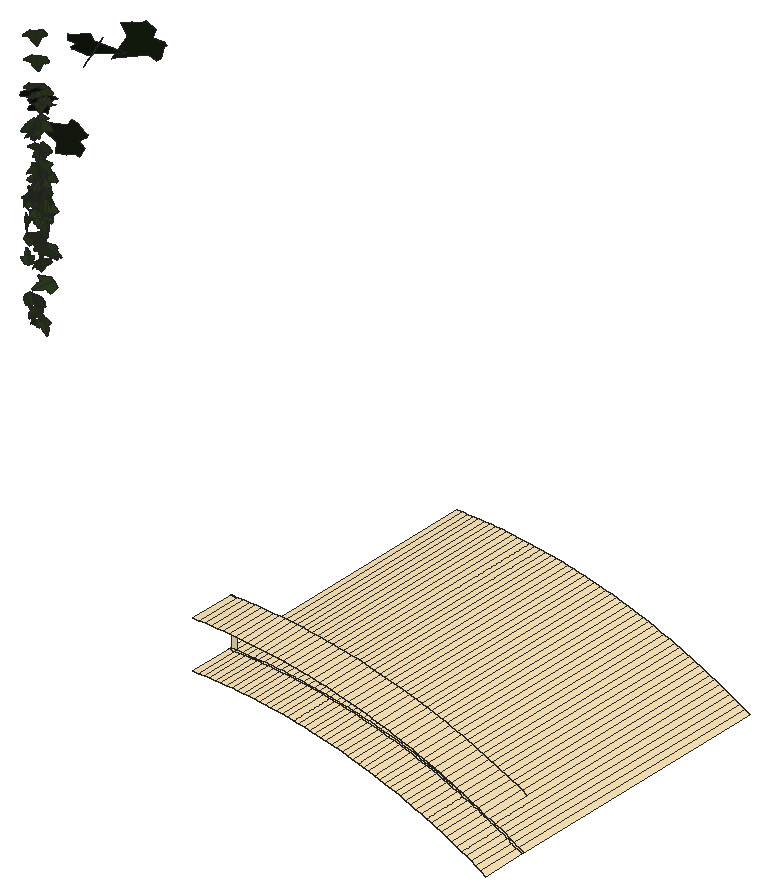
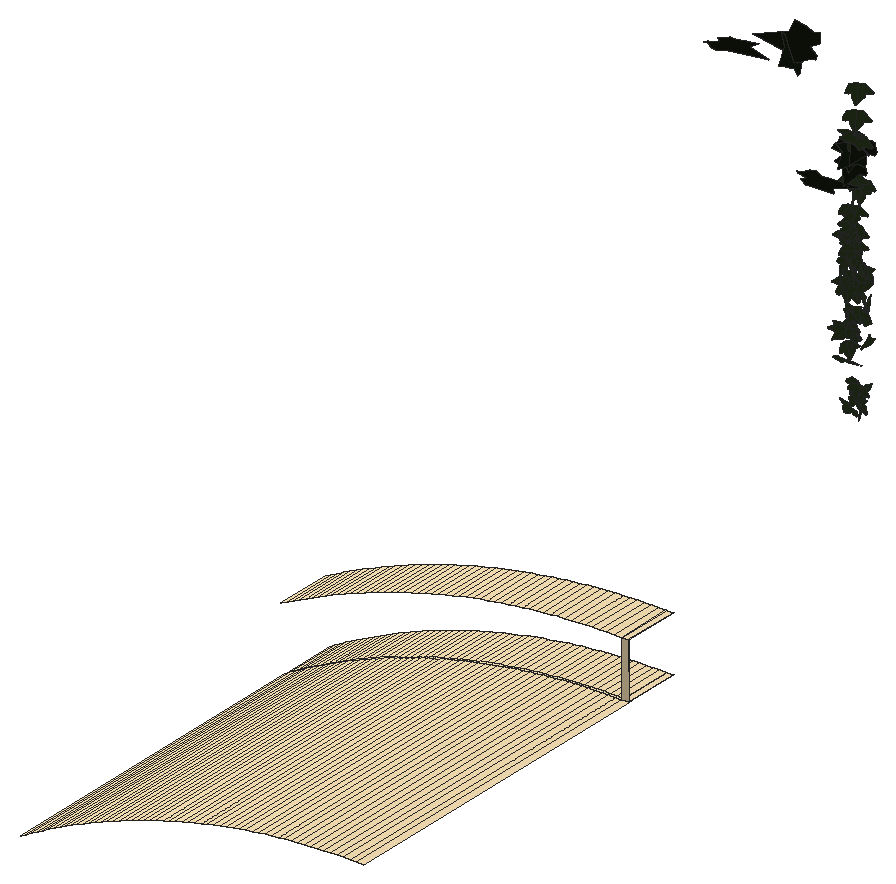
# SketchUp Ruby script. Lengths in inches.
U = 1.inch
M = Sketchup.active_model
def pt(a) = Geom::Point3d.new(a.map { |v| v * U })
def face(e, loops, mat)
  f = e.add_face(loops[0].map { |a| pt(a) })
  loops[1..].each { |l| e.add_face(l.map { |a| pt(a) }).erase! }
  f.material = f.back_material = mat if mat
  f
end
# faces: each face lists its corners as indices into pts; further lists are holes
def faces(e, pts, list, mat = nil) = list.each { |f| face(e, (f[0].is_a?(Array) ? f : [f]).map { |l| l.map { |i| pts[i] } }, mat) }
# xy, xz, yz: faces in a plane at the given z, y or x. An outline is a flat list of corners, or four numbers for a rectangle; further outlines are holes
def ring(l) = l.size == 4 ? [[l[0], l[1]], [l[2], l[1]], [l[2], l[3]], [l[0], l[3]]] : l.each_slice(2).to_a
def flat(e, list, mat, &to3) = list.each { |f| face(e, (f[0].is_a?(Array) ? f : [f]).map { |l| ring(l).map { |u, v| to3.(u, v) } }, mat) }
def xy(e, z, list, mat = nil) = flat(e, list, mat) { |x, y| [x, y, z] }
def xz(e, y, list, mat = nil) = flat(e, list, mat) { |x, z| [x, y, z] }
def yz(e, x, list, mat = nil) = flat(e, list, mat) { |y, z| [x, y, z] }
def lines(e, pts, list) = list.each { |a, b| e.add_line(pt(pts[a]), pt(pts[b])) }
# prism: a flat outline (further loops are holes) pulled along v
def prism(e, loops, v, mat = nil)
  f = face(e, loops, mat); d = Geom::Vector3d.new(v.map { |x| x * U })
  f.pushpull(f.normal.samedirection?(d) ? d.length : -d.length)
end
def box(e, o, s, mat = nil) = prism(e, [[o, [o[0] + s[0], o[1], o[2]], [o[0] + s[0], o[1] + s[1], o[2]], [o[0], o[1] + s[1], o[2]]]], [0, 0, s[2]], mat)
def at(x, y, z, deg = 0) = Geom::Transformation.translation(pt([x, y, z])) * Geom::Transformation.rotation(ORIGIN, Z_AXIS, deg.degrees)
def axes(o, x, y, z) = Geom::Transformation.new([*x, 0, *y, 0, *z, 0, *pt(o).to_a, 1])
def part(name) = M.definitions.add(name)
# library, detail: a bought-in or finely detailed component or shape, given as its bounding box
def library(name, o, s) = part(name).tap { |d| box(d.entities, o, s) }
def detail(e, o, s) = box(e.add_group.entities, o, s)
def put(e, d, t, mat = nil) = e.add_instance(d, t).tap { |i| i.material = mat if mat }
def group(e, t, mat = nil) = e.add_group.tap { |g| g.transformation = t; g.material = mat if mat }.entities
root = M.entities
M.materials.add("1026 AP 7946 SUNNY SIDE UP").color = [254, 231, 186]
M.materials.add("efeu1").color = [18, 25, 13]
M.materials.add("efeu2").color = [43, 57, 29]
c1 = part("ivyleaf_10")
p = [[0,0.5,-0.03],[-0.0625,2.02,-0.43],[-0.19,2.01,-0.46],[-0.54,1.05,-0.29],[-0.52,0.625,-0.18],[-0.83,0.76,-0.28],
  [-1.16,0.64,-0.33],[-1.15,0.33,-0.24],[-0.77,-0.39,0.02],[-0.3,-0.51,0.16],[0.04,-0.48,0.23],[-0.02,2.01,-0.4375],
  [-0.06,2.01,-0.43],[0.04,-0.49,0.23],[0.67,-0.49,0.14],[1.38,0.36,-0.2],[1.375,0.51,-0.24],[0.81,0.65,-0.19],
  [0.62,0.59,-0.15],[0.6,1.09,-0.28],[0.5,1.23,-0.31]]
faces(c1.entities,p,[[0,1,2,3,4,5,6,7,8,9,10],[11,12,0,13,14,15,16,17,18,19,20]],"efeu2")
c2 = part("ivyleaf_9")
p = [[1.54,2.16,1.25],[1.36,2.04,1.19],[-0.21,0.99,0.68],[-0.71,1.11,0.82],[-0.85,0.86,0.67],[-0.8,0.17,0.21],
  [-0.9,-0.01,0.1],[-0.67,-0.16,-0.02],[-0.08,-0.08,-0.05],[-0.03,-0.6,-0.4],[0.65,-0.88,-0.66],[0.83,-0.6,-0.49],
  [1.29,-0.42,-0.43],[1.8125,-0.07,-0.26],[1.21,0.44,0.15]]
faces(c2.entities,p,[[0,1,2,3,4,5,6,7,8,9,10,11,12,13,14]],"efeu1")
xy(root,245.999,[[153.231,213.099,153.236,215],[153.231,215,153.236,215.099]],"1026 AP 7946 SUNNY SIDE UP")
xy(root,246,[[152.978,213.099,153,215,153.002,215,152.981,213.099],[153,215,153,215.099,153.004,215.099,153.002,215],[153,215,153.002,215.099,153.004,215.099,153.002,215]],"1026 AP 7946 SUNNY SIDE UP")
xy(root,247.999,[[153.241,213.099,153.255,215.099]],"1026 AP 7946 SUNNY SIDE UP")
xy(root,248,[[152.988,213.099,153.012,215.099,153.004,215.1,152.981,213.1]],"1026 AP 7946 SUNNY SIDE UP")
xz(root,215.099,[[153.231,245.999,153.004,246,153.012,248,153.241,247.999]],"1026 AP 7946 SUNNY SIDE UP")
p = [[165.136,213.099,242.706],[165.136,215,242.706],[165.338,215,242.585],[165.338,213.099,242.585],[165.136,215.099,242.706],[165.338,215.099,242.585],
  [165.338,227,242.585],[165.136,227,242.706],[164.932,213.099,242.824],[164.932,215,242.824],[164.932,215.099,242.824],[164.932,227,242.824],
  [164.727,213.099,242.94],[164.727,215,242.94],[164.727,215.099,242.94],[164.727,227,242.94],[164.521,213.099,243.054],[164.521,215,243.054],
  [164.521,215.099,243.054],[164.521,227,243.054],[164.314,213.099,243.166],[164.314,215,243.166],[164.314,215.099,243.166],[164.314,227,243.166],
  [164.105,213.099,243.276],[164.105,215,243.276],[164.105,215.099,243.276],[164.105,227,243.276],[163.896,213.099,243.384],[163.896,215,243.384],
  [163.896,215.099,243.384],[163.896,227,243.384],[163.685,213.099,243.49],[163.685,215,243.49],[163.685,215.099,243.49],[163.685,227,243.49],
  [163.474,213.099,243.594],[163.474,215,243.594],[163.474,215.099,243.594],[163.474,227,243.594],[163.261,213.099,243.696],[163.261,215,243.696],
  [163.261,215.099,243.696],[163.261,227,243.696],[163.048,213.099,243.795],[163.048,215,243.795],[163.048,215.099,243.795],[163.048,227,243.795],
  [162.833,213.099,243.893],[162.833,215,243.893],[162.833,215.099,243.893],[162.833,227,243.893],[162.618,213.099,243.989],[162.618,215,243.989],
  [162.618,215.099,243.989],[162.618,227,243.989],[162.402,213.099,244.082],[162.402,215,244.082],[162.402,215.099,244.082],[162.402,227,244.082],
  [162.184,213.099,244.173],[162.184,215,244.173],[162.184,215.099,244.173],[162.184,227,244.173],[161.966,213.099,244.262],[161.966,215,244.262],
  [161.966,215.099,244.262],[161.966,227,244.262],[161.527,213.099,244.434],[161.527,215,244.434],[161.747,215,244.349],[161.747,213.099,244.349],
  [161.527,215.099,244.434],[161.747,215.099,244.349],[161.747,227,244.349],[161.527,227,244.434],[161.307,213.099,244.517],[161.307,215,244.517],
  [161.307,215.099,244.517],[161.307,227,244.517],[161.085,213.099,244.597],[161.085,215,244.597],[161.085,215.099,244.597],[161.085,227,244.597],
  [160.863,213.099,244.675],[160.863,215,244.675],[160.863,215.099,244.675],[160.863,227,244.675],[160.64,213.099,244.751],[160.64,215,244.751],
  [160.64,215.099,244.751],[160.64,227,244.751],[160.192,213.099,244.897],[160.192,215,244.897],[160.416,215,244.825],[160.416,213.099,244.825],
  [165.481,213.099,244.809],[165.481,215.099,244.809],[165.256,215.099,244.93],[165.256,213.099,244.93],[160.192,215.099,244.897],[160.416,215.099,244.825],
  [160.416,227,244.825],[160.192,227,244.897],[159.967,213.099,244.967],[159.967,215,244.967],[165.031,215.099,245.049],[165.031,213.099,245.049],
  [159.967,215.099,244.967],[159.967,227,244.967],[159.515,213.099,245.099],[159.515,215,245.099],[159.741,215,245.034],[159.741,213.099,245.034],
  [164.804,215.099,245.166],[164.804,213.099,245.166],[159.515,215.099,245.099],[159.741,215.099,245.034],[159.741,227,245.034],[159.515,227,245.099],
  [159.287,213.099,245.162],[159.287,215,245.162],[159.287,215.099,245.162],[159.287,227,245.162],[158.832,213.099,245.281],[158.832,215,245.281],
  [159.06,215,245.222],[159.06,213.099,245.222],[164.576,215.099,245.281],[164.576,213.099,245.281],[158.832,215.099,245.281],[159.06,215.099,245.222],
  [159.06,227,245.222],[158.832,227,245.281],[158.373,213.099,245.391],[158.373,215,245.391],[158.603,215,245.337],[158.603,213.099,245.337],
  [164.347,215.099,245.393],[164.347,213.099,245.393],[158.373,215.099,245.391],[158.603,215.099,245.337],[158.603,227,245.337],[158.373,227,245.391],
  [157.913,213.099,245.492],[157.913,215,245.492],[158.143,215,245.442],[158.143,213.099,245.442],[164.116,215.099,245.504],[164.116,213.099,245.504],
  [157.913,215.099,245.492],[158.143,215.099,245.442],[158.143,227,245.442],[157.913,227,245.492],[157.451,213.099,245.584],[157.451,215,245.584],
  [157.682,215,245.539],[157.682,213.099,245.539],[163.885,215.099,245.612],[163.885,213.099,245.612],[157.451,215.099,245.584],[157.682,215.099,245.539],
  [157.682,227,245.539],[157.451,227,245.584],[156.987,213.099,245.667],[156.987,215,245.667],[157.219,215,245.626],[157.219,213.099,245.626],
  [163.653,215.099,245.717],[163.653,213.099,245.717],[156.987,215.099,245.667],[157.219,215.099,245.626],[157.219,227,245.626],[156.987,227,245.667],
  [156.288,213.099,245.774],[156.288,215,245.774],[156.522,215,245.74],[156.522,213.099,245.74],[156.754,215,245.705],[156.754,213.099,245.705],
  [163.419,215.099,245.821],[163.419,213.099,245.821],[156.288,215.099,245.774],[156.522,215.099,245.74],[156.754,215.099,245.705],[156.522,227,245.74],
  [156.288,227,245.774],[156.754,227,245.705],[155.587,213.099,245.86],[155.587,215,245.86],[155.821,215,245.834],[155.821,213.099,245.834],
  [156.055,215,245.805],[156.055,213.099,245.805],[163.185,215.099,245.922],[163.185,213.099,245.922],[155.587,215.099,245.86],[155.821,215.099,245.834],
  [156.055,215.099,245.805],[155.821,227,245.834],[155.587,227,245.86],[156.055,227,245.805],[154.413,213.099,245.958],[154.413,215,245.958],
  [154.648,215,245.943],[154.648,213.099,245.943],[154.883,215,245.926],[154.883,213.099,245.926],[155.118,215,245.906],[155.118,213.099,245.906],
  [155.352,215,245.884],[155.352,213.099,245.884],[162.95,215.099,246.021],[162.95,213.099,246.021],[154.413,215.099,245.958],[154.648,215.099,245.943],
  [154.883,215.099,245.926],[155.118,215.099,245.906],[155.352,215.099,245.884],[154.648,227,245.943],[154.413,227,245.958],[154.883,227,245.926],
  [155.118,227,245.906],[155.352,227,245.884],[152.981,213.099,246],[153.002,215,246],[153.231,215,245.999],[153.231,213.099,245.999],
  [153.236,213.099,245.999],[153.236,215,245.999],[153.471,215,245.995],[153.471,213.099,245.995],[153.707,215,245.99],[153.707,213.099,245.99],
  [153.942,215,245.981],[153.942,213.099,245.981],[154.178,215,245.971],[154.178,213.099,245.971],[162.713,215.099,246.117],[162.713,213.099,246.117],
  [153.004,215.099,246],[153.231,215.099,245.999],[153.236,215.099,245.999],[153.471,215.099,245.995],[153.707,215.099,245.99],[153.942,215.099,245.981],
  [154.178,215.099,245.971],[153.012,215.099,248],[153.002,215.099,246],[153.004,215.1,248],[153.236,227,245.999],[153,215.099,246],
  [153,227,246],[153.471,227,245.995],[153.707,227,245.99],[153.942,227,245.981],[154.178,227,245.971],[162.476,215.099,246.212],
  [162.476,213.099,246.212],[162.238,215.099,246.303],[162.238,213.099,246.303],[161.999,215.099,246.393],[161.999,213.099,246.393],[161.759,215.099,246.48],
  [161.759,213.099,246.48],[161.518,215.099,246.565],[161.518,213.099,246.565],[161.277,213.099,246.647],[161.277,215.099,246.647],[161.034,215.099,246.727],
  [161.034,213.099,246.727],[160.791,215.099,246.805],[160.791,213.099,246.805],[160.547,215.099,246.88],[160.547,213.099,246.88],[160.303,215.099,246.953],
  [160.303,213.099,246.953],[160.057,213.099,247.024],[160.057,215.099,247.024],[159.811,215.099,247.092],[159.811,213.099,247.092],[159.565,215.099,247.158],
  [159.565,213.099,247.158],[159.317,213.099,247.221],[159.317,215.099,247.221],[159.07,215.099,247.282],[159.07,213.099,247.282],[158.821,213.099,247.34],
  [158.821,215.099,247.34],[158.572,215.099,247.396],[158.572,213.099,247.396],[158.322,213.099,247.449],[158.322,215.099,247.449],[158.072,215.099,247.5],
  [158.072,213.099,247.5],[157.822,213.099,247.549],[157.822,215.099,247.549],[157.571,215.099,247.595],[157.571,213.099,247.595],[157.319,213.099,247.639],
  [157.319,215.099,247.639],[157.067,215.099,247.68],[157.067,213.099,247.68],[156.815,213.099,247.719],[156.815,215.099,247.719],[156.5625,215.099,247.755],
  [156.5625,213.099,247.755],[155.802,213.099,247.849],[155.802,215.099,247.849],[155.548,215.099,247.875],[155.548,213.099,247.875],[156.056,213.099,247.82],
  [156.056,215.099,247.82],[156.309,213.099,247.789],[156.309,215.099,247.789],[154.785,213.099,247.939],[154.785,215.099,247.939],[154.531,215.099,247.955],
  [154.531,213.099,247.955],[155.04,213.099,247.92],[155.04,215.099,247.92],[155.294,213.099,247.899],[155.294,215.099,247.899],[153.241,213.099,247.999],
  [153.241,215.099,247.999],[152.988,213.099,248],[153.51,213.099,247.995],[153.51,215.099,247.995],[153.255,215.099,247.999],[153.255,213.099,247.999],
  [153.766,213.099,247.989],[153.766,215.099,247.989],[154.021,213.099,247.98],[154.021,215.099,247.98],[154.276,213.099,247.969],[154.276,215.099,247.969]]
faces(root,p,[[0,1,2,3],[1,4,5,2],[6,5,4,7],[8,9,1,0],[9,10,4,1],[7,4,10,11],[12,13,9,8],[13,14,10,9],
  [11,10,14,15],[16,17,13,12],[17,18,14,13],[15,14,18,19],[20,21,17,16],[21,22,18,17],[19,18,22,23],[24,25,21,20],
  [25,26,22,21],[23,22,26,27],[28,29,25,24],[29,30,26,25],[27,26,30,31],[32,33,29,28],[33,34,30,29],[31,30,34,35],
  [36,37,33,32],[37,38,34,33],[35,34,38,39],[40,41,37,36],[41,42,38,37],[39,38,42,43],[44,45,41,40],[45,46,42,41],
  [43,42,46,47],[48,49,45,44],[49,50,46,45],[47,46,50,51],[52,53,49,48],[53,54,50,49],[51,50,54,55],[56,57,53,52],
  [57,58,54,53],[55,54,58,59],[60,61,57,56],[61,62,58,57],[59,58,62,63],[64,65,61,60],[65,66,62,61],[63,62,66,67],
  [68,69,70,71],[71,70,65,64],[69,72,73,70],[70,73,66,65],[74,73,72,75],[67,66,73,74],[76,77,69,68],[77,78,72,69],
  [75,72,78,79],[80,81,77,76],[81,82,78,77],[79,78,82,83],[84,85,81,80],[85,86,82,81],[83,82,86,87],[88,89,85,84],
  [89,90,86,85],[87,86,90,91],[92,93,94,95],[95,94,89,88],[96,97,98,99],[93,100,101,94],[94,101,90,89],[102,101,100,103],
  [91,90,101,102],[104,105,93,92],[99,98,106,107],[105,108,100,93],[103,100,108,109],[110,111,112,113],[113,112,105,104],[107,106,114,115],
  [111,116,117,112],[112,117,108,105],[118,117,116,119],[109,108,117,118],[120,121,111,110],[121,122,116,111],[119,116,122,123],[124,125,126,127],
  [127,126,121,120],[115,114,128,129],[125,130,131,126],[126,131,122,121],[132,131,130,133],[123,122,131,132],[134,135,136,137],[137,136,125,124],
  [129,128,138,139],[135,140,141,136],[136,141,130,125],[142,141,140,143],[133,130,141,142],[144,145,146,147],[147,146,135,134],[139,138,148,149],
  [145,150,151,146],[146,151,140,135],[152,151,150,153],[143,140,151,152],[154,155,156,157],[157,156,145,144],[149,148,158,159],[155,160,161,156],
  [156,161,150,145],[162,161,160,163],[153,150,161,162],[164,165,166,167],[167,166,155,154],[159,158,168,169],[165,170,171,166],[166,171,160,155],
  [172,171,170,173],[163,160,171,172],[174,175,176,177],[177,176,178,179],[179,178,165,164],[169,168,180,181],[175,182,183,176],[176,183,184,178],
  [178,184,170,165],[185,183,182,186],[187,184,183,185],[173,170,184,187],[188,189,190,191],[191,190,192,193],[193,192,175,174],[181,180,194,195],
  [189,196,197,190],[190,197,198,192],[192,198,182,175],[199,197,196,200],[201,198,197,199],[186,182,198,201],[202,203,204,205],[205,204,206,207],
  [207,206,208,209],[209,208,210,211],[211,210,189,188],[195,194,212,213],[203,214,215,204],[204,215,216,206],[206,216,217,208],[208,217,218,210],
  [210,218,196,189],[219,215,214,220],[221,216,215,219],[222,217,216,221],[223,218,217,222],[200,196,218,223],[224,225,226,227],[228,229,230,231],
  [231,230,232,233],[233,232,234,235],[235,234,236,237],[237,236,203,202],[213,212,238,239],[240,241,226,225],[229,242,243,230],[230,243,244,232],
  [232,244,245,234],[234,245,246,236],[236,246,214,203],[247,240,248,249],[250,242,241,240,248,251,252],[253,243,242,250],[254,244,243,253],[255,245,244,254],
  [256,246,245,255],[220,214,246,256],[239,238,257,258],[258,257,259,260],[260,259,261,262],[262,261,263,264],[264,263,265,266],[267,268,269,270],
  [266,265,268,267],[270,269,271,272],[272,271,273,274],[274,273,275,276],[277,278,279,280],[276,275,278,277],[280,279,281,282],[283,284,285,286],
  [282,281,284,283],[287,288,289,290],[286,285,288,287],[291,292,293,294],[290,289,292,291],[295,296,297,298],[294,293,296,295],[299,300,301,302],
  [298,297,300,299],[303,304,305,306],[302,301,304,303],[307,308,309,310],[311,312,308,307],[313,314,312,311],[306,305,314,313],[315,316,317,318],
  [319,320,316,315],[321,322,320,319],[310,309,322,321],[323,324,247,325],[326,327,328,329],[330,331,327,326],[332,333,331,330],[334,335,333,332],
  [318,317,335,334]],"1026 AP 7946 SUNNY SIDE UP")
put(root,c1,axes([145.875,213.31,261.2],[0.05616,0.14878,0.14238],[0.01858,0.13771,-0.15602],[-0.31786,0.03434,0.01604]),"1026 AP 7946 SUNNY SIDE UP")
put(root,c1,axes([145.97,213.08,260.51],[0.04021,-0.03429,-0.22157],[0.01532,0.21632,-0.0331],[0.34181,-0.00566,0.02755]),"1026 AP 7946 SUNNY SIDE UP")
put(root,c1,axes([146,213.22,261.48],[-0.01385,-0.1985,0.07269],[-0.00757,-0.07154,-0.20511],[0.33177,-0.00992,-0.00165]),"1026 AP 7946 SUNNY SIDE UP")
put(root,c1,axes([146,213.34,261.64],[0.02016,-0.20459,-0.01266],[-0.00594,0.01091,-0.21109],[0.32212,0.01301,-0.0031]),"1026 AP 7946 SUNNY SIDE UP")
put(root,c1,axes([146.02,213.31,260.72],[0.11865,-0.18058,-0.05731],[-0.04723,0.04656,-0.20112],[0.29286,0.08067,-0.00922]),"1026 AP 7946 SUNNY SIDE UP")
put(root,c1,axes([145.99,213.625,261.41],[0.12895,-0.14013,0.12572],[-0.08622,0.11011,0.16777],[-0.28004,-0.09843,0.00624]),"1026 AP 7946 SUNNY SIDE UP")
put(root,c1,axes([146.05,213.1,259.06],[0.03463,0.20193,-0.04329],[-0.01225,0.0442,0.20914],[0.32446,-0.01988,0.01252]),"1026 AP 7946 SUNNY SIDE UP")
put(root,c1,axes([146.0625,213.48,267.52],[-0.25717,-0.18381,-0.01709],[0.043,-0.00362,-0.2524],[0.28685,-0.16425,0.02252]),"1026 AP 7946 SUNNY SIDE UP")
put(root,c1,axes([146.1,213.24,261.625],[-0.27434,0.11876,0.04143],[-0.06812,0.00634,-0.21653],[-0.18465,-0.17878,0.01833]),"1026 AP 7946 SUNNY SIDE UP")
put(root,c1,axes([146.02,213.09,257.71],[0.00938,0.20748,0.04155],[-0.0202,0.03945,-0.21313],[-0.33139,0.00346,0.01417]),"1026 AP 7946 SUNNY SIDE UP")
put(root,c1,axes([146.16,213.45,266.6],[-0.29699,-0.14844,-0.0074],[0.02684,-0.0115,-0.24672],[0.23207,-0.18863,0.01907]),"1026 AP 7946 SUNNY SIDE UP")
put(root,c1,axes([145.99,213.64,261.5625],[0.25664,0.0746,0.10249],[0.14758,0.03271,-0.18449],[-0.12745,0.1881,-0.00726]),"1026 AP 7946 SUNNY SIDE UP")
put(root,c1,axes([146.2,213.26,257.69],[-0.32008,0.02802,-0.00049],[-0.00324,-0.01962,-0.21082],[-0.04395,-0.20262,0.01912]),"1026 AP 7946 SUNNY SIDE UP")
put(root,c1,axes([146.21,213.14,264.0625],[-0.04075,-0.23488,-0.07701],[0.05294,0.06975,-0.24171],[0.38332,-0.0346,0.02519]),"1026 AP 7946 SUNNY SIDE UP")
put(root,c1,axes([146.39,213.14,257.23],[-0.25575,0.0259,0.12607],[-0.19645,-0.03528,-0.16378],[0.00153,-0.20037,0.04391]),"1026 AP 7946 SUNNY SIDE UP")
put(root,c2,axes([146.17,213.04,265.55],[0.24851,0.20325,0.03095],[0.04687,0.01336,-0.2647],[-0.31939,0.16011,-0.01476]),"1026 AP 7946 SUNNY SIDE UP")
put(root,c1,axes([146.21,213.13,264.22],[-0.2365,-0.18539,-0.07579],[0.12986,0.02458,-0.24107],[0.2848,-0.16515,0.04699]),"1026 AP 7946 SUNNY SIDE UP")
put(root,c1,axes([146.24,213.12,257.0625],[0.09709,-0.19108,-0.05805],[0.04788,0.06626,-0.2006],[0.30909,0.04976,0.0493]),"1026 AP 7946 SUNNY SIDE UP")
put(root,c1,axes([146.03,213.14,259.95],[0.10748,0.00075,0.19926],[0.29747,0.04246,-0.0688],[-0.06334,0.2007,0.01503]),"1026 AP 7946 SUNNY SIDE UP")
put(root,c1,axes([146.34,213.37,259.73],[0.21683,-0.14191,-0.07285],[-0.08649,0.04395,-0.20341],[0.23323,0.14823,-0.0077]),"1026 AP 7946 SUNNY SIDE UP")
put(root,c1,axes([146.25,213.67,261.32],[-0.04946,-0.18283,-0.08532],[0.11365,0.06684,-0.18219],[0.29371,-0.05665,0.05614]),"1026 AP 7946 SUNNY SIDE UP")
put(root,c1,axes([146.3,213.23,262.63],[-0.13376,-0.21694,-0.04271],[0.0821,0.0221,-0.23637],[0.33708,-0.09147,0.04062]),"1026 AP 7946 SUNNY SIDE UP")
put(root,c1,axes([146.45,213.3,260.87],[-0.29052,-0.06558,0.09691],[-0.12381,-0.05809,-0.20059],[0.13175,-0.1992,0.02519]),"1026 AP 7946 SUNNY SIDE UP")
put(root,c2,axes([146.29,213.31,264.9375],[0.2185,0.19989,0.01727],[0.02779,0.00673,-0.25051],[-0.31404,0.13967,-0.01015]),"1026 AP 7946 SUNNY SIDE UP")
put(root,c1,axes([146.3,213.22,265.7],[-0.35897,-0.09349,-0.05141],[0.08568,-0.00336,-0.25303],[0.14246,-0.23355,0.02264]),"1026 AP 7946 SUNNY SIDE UP")
put(root,c1,axes([146.31,213.36,262.43],[-0.28081,0.09711,-0.05456],[0.01604,-0.08663,-0.19754],[-0.17361,-0.16508,0.07]),"1026 AP 7946 SUNNY SIDE UP")
put(root,c1,axes([146.36,213.38,259.74],[-0.29777,0.09207,0.00729],[-0.03202,-0.02709,-0.21436],[-0.14156,-0.18754,0.03316]),"1026 AP 7946 SUNNY SIDE UP")
put(root,c1,axes([146.39,213.34,262.2],[-0.03509,-0.20379,0.09763],[-0.00695,-0.09598,-0.21168],[0.35409,-0.02208,0.00552]),"1026 AP 7946 SUNNY SIDE UP")
put(root,c1,axes([146.41,213.34,260.1],[-0.04788,-0.17764,0.1165],[-0.02178,-0.11335,-0.18628],[0.33126,-0.03313,0.00459]),"1026 AP 7946 SUNNY SIDE UP")
put(root,c1,axes([146.42,213.3,263.4],[-0.32663,-0.10436,0.01521],[-0.00928,-0.02237,-0.23895],[0.16561,-0.20709,0.01661]),"1026 AP 7946 SUNNY SIDE UP")
put(root,c1,axes([146.36,213.3,263.26],[0.09561,0.22066,-0.05651],[-0.0509,-0.04911,-0.23538],[-0.35437,0.06659,0.01856]),"1026 AP 7946 SUNNY SIDE UP")
put(root,c2,axes([146.31,213.22,265.24],[0.26542,0.16148,0.09072],[0.04949,0.09118,-0.23632],[-0.28425,0.16665,0.04357]),"1026 AP 7946 SUNNY SIDE UP")
put(root,c1,axes([146.42,213.24,264.34],[0.33969,0.0994,-0.05962],[-0.09173,-0.01281,-0.24473],[-0.15638,0.22343,0.01406]),"1026 AP 7946 SUNNY SIDE UP")
put(root,c1,axes([146.375,213.38,262.3],[-0.00059,-0.1665,0.15589],[0.00035,0.15226,0.17242],[-0.35477,0.00043,-0.00009]),"1026 AP 7946 SUNNY SIDE UP")
put(root,c1,axes([146.47,213.44,259.06],[-0.15597,-0.17456,0.03025],[-0.00638,-0.03254,-0.20663],[0.27852,-0.0985,0.01221]),"1026 AP 7946 SUNNY SIDE UP")
put(root,c1,axes([146.42,213.2,264.48],[0.03117,0.23648,0.05797],[-0.0525,0.05724,-0.24114],[-0.37811,0.01155,0.03826]),"1026 AP 7946 SUNNY SIDE UP")
put(root,c1,axes([146.51,213.28,261.96],[-0.35162,0.02906,0.03794],[-0.06484,-0.03786,-0.2284],[-0.03474,-0.22342,0.04227]),"1026 AP 7946 SUNNY SIDE UP")
put(root,c1,axes([146.42,213.51,260.08],[-0.15773,0.14679,-0.1025],[0.00143,-0.11478,-0.17459],[-0.27957,-0.0834,0.05694]),"1026 AP 7946 SUNNY SIDE UP")
put(root,c1,axes([146.48,213.1875,265.35],[-0.39161,-0.03642,0.00712],[0.00713,-0.07783,-0.24711],[0.05791,-0.23668,0.0786]),"1026 AP 7946 SUNNY SIDE UP")
put(root,c1,axes([146.44,213.16,259.19],[0.00811,-0.21304,-0.05971],[0.05424,0.05685,-0.21629],[0.3424,-0.00396,0.03567]),"1026 AP 7946 SUNNY SIDE UP")
put(root,c1,axes([146.44,213.19,262.23],[0.35946,0.03264,-0.03796],[-0.05706,-0.00781,-0.23792],[-0.05261,0.23145,-0.0013]),"1026 AP 7946 SUNNY SIDE UP")
put(root,c1,axes([146.43,213.13,257.71],[-0.27001,0.10187,-0.04669],[0.04555,-0.04069,-0.20492],[-0.16968,-0.17302,0.01928]),"1026 AP 7946 SUNNY SIDE UP")
put(root,c1,axes([146.42,213.26,262.59],[-0.06583,0.21661,-0.04739],[0.00284,-0.04773,-0.22744],[-0.34858,-0.0413,0.0071]),"1026 AP 7946 SUNNY SIDE UP")
put(root,c1,axes([146.47,213.29,261.78],[0.08028,-0.21224,0.05501],[0.02839,-0.0518,-0.22512],[0.34342,0.0539,0.00575]),"1026 AP 7946 SUNNY SIDE UP")
put(root,c1,axes([146.51,213.43,260.9],[-0.21996,-0.15754,0.00894],[0.00594,-0.01613,-0.21669],[0.24811,-0.13929,0.01312]),"1026 AP 7946 SUNNY SIDE UP")
put(root,c1,axes([146.43,213.27,260.89],[0.29508,0.11119,-0.02455],[-0.01977,-0.02664,-0.22424],[-0.17793,0.18737,-0.0158]),"1026 AP 7946 SUNNY SIDE UP")
put(root,c2,axes([146.53,213.17,265.34],[0.16264,0.22699,-0.03023],[-0.00743,-0.03149,-0.257],[-0.36008,0.10318,-0.00835]),"1026 AP 7946 SUNNY SIDE UP")
put(root,c1,axes([146.49,213.27,263.45],[-0.07052,0.23336,-0.01381],[-0.01605,-0.01693,-0.24453],[-0.36731,-0.04407,0.01333]),"1026 AP 7946 SUNNY SIDE UP")
put(root,c1,axes([146.51,213.32,261.3125],[0.04293,0.21322,-0.05919],[-0.04408,-0.0553,-0.22081],[-0.34493,0.0336,0.02085]),"1026 AP 7946 SUNNY SIDE UP")
put(root,c1,axes([146.43,213.22,262.8125],[-0.27527,-0.08418,-0.14038],[0.21711,0.02162,-0.19707],[0.12639,-0.2205,0.03278]),"1026 AP 7946 SUNNY SIDE UP")
put(root,c1,axes([146.43,213.18,265.6875],[0.36974,0.03098,0.07823],[0.11936,0.00365,-0.24424],[-0.04814,0.24702,-0.00473]),"1026 AP 7946 SUNNY SIDE UP")
put(root,c1,axes([146.53,213.4,260.41],[0.24266,-0.12087,0.06597],[0.06707,-0.05029,-0.20182],[0.2049,0.15961,-0.01206]),"1026 AP 7946 SUNNY SIDE UP")
put(root,c1,axes([146.5,213.33,261],[0.13588,0.17884,0.10163],[0.06376,0.08884,-0.2041],[-0.31399,0.09544,0.00254]),"1026 AP 7946 SUNNY SIDE UP")
put(root,c1,axes([146.57,213.4,261.16],[0.21694,0.16374,-0.03897],[-0.02415,-0.03766,-0.22044],[-0.26348,0.13827,-0.01188]),"1026 AP 7946 SUNNY SIDE UP")
put(root,c1,axes([146.82,213.26,258.42],[-0.31117,0.10295,0.1091],[-0.21136,-0.19834,-0.06162],[0.09463,-0.10447,0.2211]),"1026 AP 7946 SUNNY SIDE UP")
put(root,c1,axes([146.64,213.37,261.66],[-0.24451,0.15744,0.00569],[-0.01896,-0.00541,-0.22764],[-0.24694,-0.15548,0.01184]),"1026 AP 7946 SUNNY SIDE UP")
put(root,c1,axes([146.54,213.45,259.52],[-0.21214,-0.09495,-0.12527],[0.18091,0.04463,-0.16789],[0.16061,-0.17568,0.02366]),"1026 AP 7946 SUNNY SIDE UP")
put(root,c1,axes([146.64,213.3,262.47],[0.35397,0.02675,-0.025],[-0.03514,-0.01842,-0.2331],[-0.04483,0.22569,-0.01471]),"1026 AP 7946 SUNNY SIDE UP")
put(root,c1,axes([146.54,213.45,259.6],[-0.15697,-0.0234,-0.18352],[0.28081,-0.03392,-0.09878],[-0.02907,-0.20125,0.03676]),"1026 AP 7946 SUNNY SIDE UP")
put(root,c1,axes([146.57,213.2,256.92],[0.25591,-0.02146,0.12574],[0.18383,-0.04083,-0.16807],[0.06519,0.19937,-0.01966]),"1026 AP 7946 SUNNY SIDE UP")
put(root,c2,axes([147.74,213.54,264.03],[-0.36713,-0.18715,-0.26169],[-0.34903,-0.1253,0.30584],[-0.35069,0.32063,-0.03043]),"1026 AP 7946 SUNNY SIDE UP")
put(root,c2,axes([148.57,213.16,267.59],[0.0793,0.15776,0.35804],[0.13796,0.33546,-0.16846],[-0.58275,0.10088,0.00884]),"1026 AP 7946 SUNNY SIDE UP")
put(root,c2,axes([148.12,213.14,267.97],[0.32658,0.00337,0.33115],[0.50542,-0.00511,-0.21395],[0.00387,0.38266,-0.00354]),"1026 AP 7946 SUNNY SIDE UP")
put(root,c2,axes([149.95,214.69,268.14],[-0.59395,-0.16999,0.14103],[-0.16873,-0.09583,-0.42518],[0.29995,-0.39052,0.04009]),"1026 AP 7946 SUNNY SIDE UP")
